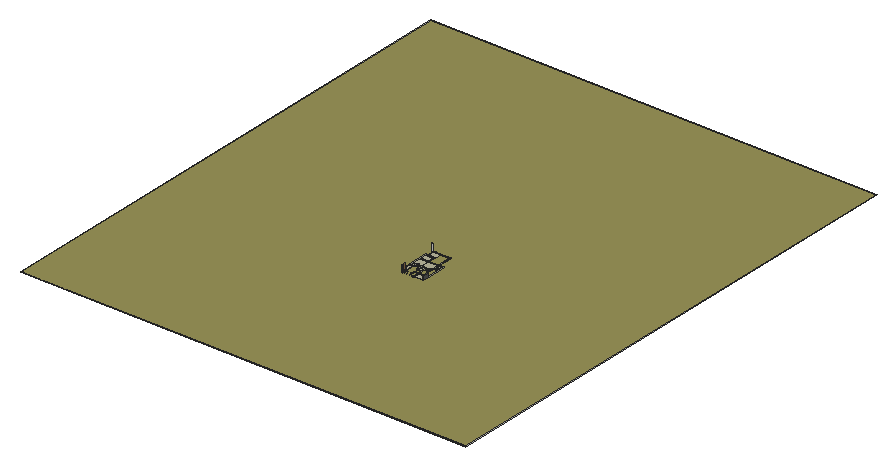
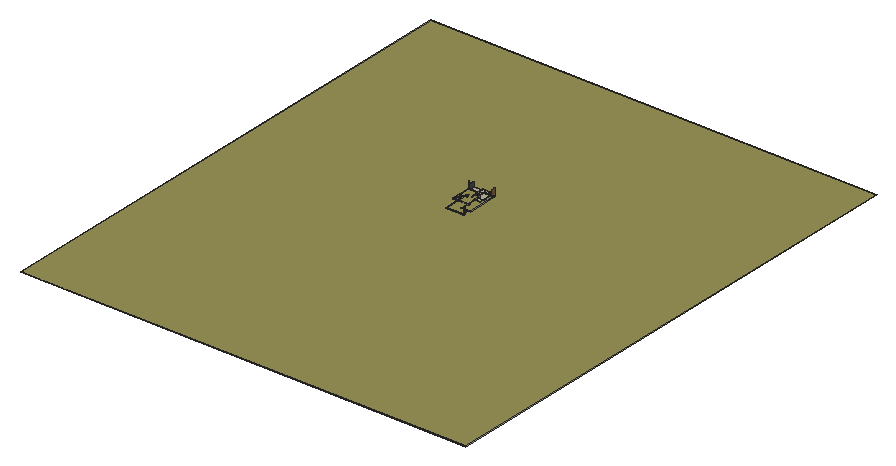
# SketchUp Ruby script. Lengths in inches.
U = 1.inch
M = Sketchup.active_model
def pt(a) = Geom::Point3d.new(a.map { |v| v * U })
def face(e, loops, mat)
  f = e.add_face(loops[0].map { |a| pt(a) })
  loops[1..].each { |l| e.add_face(l.map { |a| pt(a) }).erase! }
  f.material = f.back_material = mat if mat
  f
end
# faces: each face lists its corners as indices into pts; further lists are holes
def faces(e, pts, list, mat = nil) = list.each { |f| face(e, (f[0].is_a?(Array) ? f : [f]).map { |l| l.map { |i| pts[i] } }, mat) }
# xy, xz, yz: faces in a plane at the given z, y or x. An outline is a flat list of corners, or four numbers for a rectangle; further outlines are holes
def ring(l) = l.size == 4 ? [[l[0], l[1]], [l[2], l[1]], [l[2], l[3]], [l[0], l[3]]] : l.each_slice(2).to_a
def flat(e, list, mat, &to3) = list.each { |f| face(e, (f[0].is_a?(Array) ? f : [f]).map { |l| ring(l).map { |u, v| to3.(u, v) } }, mat) }
def xy(e, z, list, mat = nil) = flat(e, list, mat) { |x, y| [x, y, z] }
def xz(e, y, list, mat = nil) = flat(e, list, mat) { |x, z| [x, y, z] }
def yz(e, x, list, mat = nil) = flat(e, list, mat) { |y, z| [x, y, z] }
def lines(e, pts, list) = list.each { |a, b| e.add_line(pt(pts[a]), pt(pts[b])) }
# prism: a flat outline (further loops are holes) pulled along v
def prism(e, loops, v, mat = nil)
  f = face(e, loops, mat); d = Geom::Vector3d.new(v.map { |x| x * U })
  f.pushpull(f.normal.samedirection?(d) ? d.length : -d.length)
end
def box(e, o, s, mat = nil) = prism(e, [[o, [o[0] + s[0], o[1], o[2]], [o[0] + s[0], o[1] + s[1], o[2]], [o[0], o[1] + s[1], o[2]]]], [0, 0, s[2]], mat)
def at(x, y, z, deg = 0) = Geom::Transformation.translation(pt([x, y, z])) * Geom::Transformation.rotation(ORIGIN, Z_AXIS, deg.degrees)
def axes(o, x, y, z) = Geom::Transformation.new([*x, 0, *y, 0, *z, 0, *pt(o).to_a, 1])
def part(name) = M.definitions.add(name)
# library, detail: a bought-in or finely detailed component or shape, given as its bounding box
def library(name, o, s) = part(name).tap { |d| box(d.entities, o, s) }
def detail(e, o, s) = box(e.add_group.entities, o, s)
def put(e, d, t, mat = nil) = e.add_instance(d, t).tap { |i| i.material = mat if mat }
def group(e, t, mat = nil) = e.add_group.tap { |g| g.transformation = t; g.material = mat if mat }.entities
root = M.entities
M.materials.add("Concrete_04_1K").color = [184, 181, 156]
M.materials.add("M06_Steel_Smoke").color = [86, 86, 86]
M.materials.add("Plywood_01_1K").color = [125, 96, 64]
M.materials.add("Soil_04_1K").color = [152, 146, 88]
M.materials.add("Wood_Floor_01_1K").color = [146, 111, 76]
xy(root,9,[[4480,3552.7,4489,3625.01],[4489,3552.7,4621.87,3625.01],[4621.87,3552.7,4625.87,3625.01],[4625.87,3552.7,4682.8125,3635.25],[4682.8125,3552.7,4700.3125,3635.25],
  [4462.07,3564.51,4462.07,3609.04,4472.4375,3609.04,4472.4375,3625.01,4480,3625.01,4480,3564.51],[4700.3125,3566.51,4861.07,3666.98],[4861.07,3566.51,4874.8125,3666.98],[4430.07,3609.04,4472.4375,3609.04,4472.4375,3639.11,4480,3639.11,4480,3645.11,4429.38,3645.11,4429.38,3639.11,4430.07,3639.11],[4472.4375,3625.01,4480,3639.11],
  [4480,3625.01,4489,3805.79],[4489,3625.01,4489,3805.79,4591.8125,3805.79,4591.8125,3746.01,4621.87,3746.01,4621.87,3625.01],[4621.87,3625.01,4625.87,3631.25],[4621.87,3631.25,4625.87,3635.25],[4621.87,3635.25,4625.87,3666.98],
  [4625.87,3635.25,4682.8125,3666.98],[4682.8125,3635.25,4700.3125,3666.98],[4420.38,3639.11,4429.38,3645.11],[4420.38,3645.11,4429.38,3800.79],[4429.38,3645.11,4480,3800.79],
  [4621.87,3666.98,4625.87,3670.98],[4625.87,3666.98,4686.8125,3670.98],[4686.8125,3666.98,4690.8125,3670.98],[4690.8125,3666.98,4870.8125,3670.98],[4870.8125,3666.98,4874.8125,3670.98],
  [4621.87,3670.98,4625.87,3750.01],[4625.87,3670.98,4686.8125,3750.01],[4686.8125,3670.98,4690.8125,3833.04],[4870.8125,3670.98,4874.8125,3833.04],[4591.8125,3746.01,4595.8125,3750.01],
  [4595.8125,3746.01,4621.87,3750.01],[4591.8125,3750.01,4595.8125,3766.09],[4595.8125,3750.01,4686.8125,3833.04],[4591.8125,3766.09,4595.8125,3833.04],[4420.38,3800.79,4429.38,3809.79],
  [4429.38,3800.79,4480,3809.79],[4480,3805.79,4489,3809.79],[4489,3805.79,4591.8125,3809.79],[4420.38,3809.79,4489,3869.04],[4489,3809.79,4591.8125,3869.04],
  [4591.8125,3833.04,4595.8125,3869.04],[4595.8125,3833.04,4778.8125,3869.04],[4778.8125,3833.04,4784.8125,3923.04],[4865.8125,3833.04,4874.8125,3923.04],[4420.38,3869.04,4489,3878.04],
  [4489,3869.04,4591.8125,3878.04],[4723.125,3869.04,4729.125,3878.04],[4729.125,3869.04,4778.8125,3878.04],[4420.38,3878.04,4586.8125,4049.04],[4586.8125,3878.04,4595.8125,4049.04],
  [4595.8125,3878.04,4595.8125,4049.04,4769.8125,4049.04,4769.8125,4040.04,4778.8125,4040.04,4778.8125,3878.04],[4778.8125,3923.04,4784.8125,3929.04],[4784.8125,3923.04,4865.8125,3929.04],[4865.8125,3923.04,4874.8125,3929.04],[4778.8125,3929.04,4784.8125,3977.04],
  [4784.8125,3929.04,4865.8125,3977.04],[4865.8125,3929.04,4874.8125,3977.04],[4778.8125,3977.04,4784.8125,3983.04],[4784.8125,3977.04,4865.8125,3983.04],[4865.8125,3977.04,4874.8125,3983.04],
  [4778.8125,3983.04,4784.8125,4040.04],[4784.8125,3983.04,4865.8125,4040.04],[4865.8125,3983.04,4874.8125,4040.04],[4769.8125,4040.04,4778.8125,4049.04],[4778.8125,4040.04,4865.8125,4049.04],
  [4865.8125,4040.04,4874.8125,4049.04],[4420.38,4049.04,4586.8125,4058.04],[4586.8125,4049.04,4595.8125,4058.04],[4769.8125,4049.04,4778.8125,4058.04],[4420.38,4058.04,4586.8125,4176.04],
  [4769.8125,4058.04,4778.8125,4328.04],[4420.38,4176.04,4586.8125,4193.04],[4454.8125,4193.04,4463.8125,4202.04],[4463.8125,4193.04,4586.8125,4202.04],[4454.8125,4202.04,4463.8125,4328.04],
  [4463.8125,4202.04,4591.8125,4328.04],[4454.8125,4328.04,4463.8125,4337.04],[4463.8125,4328.04,4591.8125,4337.04],[4591.8125,4328.04,4769.8125,4337.04],[4769.8125,4328.04,4778.8125,4337.04]],"Concrete_04_1K")
xz(root,3552.7,[[4480,9,4700.3125,15]],"Plywood_01_1K")
xz(root,3564.51,[[4462.07,9,4480,124.125]],"Wood_Floor_01_1K")
xz(root,3566.51,[[4861.07,9,4874.8125,81.29]],"M06_Steel_Smoke")
xz(root,3609.04,[[4462.07,9,4472.4375,15]],"Concrete_04_1K")
xz(root,3609.04,[[4430.07,9,4462.07,15]],"Plywood_01_1K")
xz(root,3639.11,[[4472.4375,9,4480,15]],"Concrete_04_1K")
xz(root,3639.11,[[4420.38,9,4430.07,15]],"Plywood_01_1K")
xz(root,3645.11,[[4429.38,9,4480,15]],"Concrete_04_1K")
xz(root,3666.98,[[4625.87,9,4682.8125,9,4695.7,15,4625.87,15],[4682.8125,9,4700.3125,9,4700.3125,15,4695.7,15],[4700.3125,9,4861.07,15],[4861.07,9,4874.8125,15]],"Concrete_04_1K")
xz(root,3670.98,[[4625.87,9,4686.8125,15],[4690.8125,9,4870.8125,15]],"Concrete_04_1K")
xz(root,3746.01,[[4591.8125,9,4595.8125,15],[4595.8125,9,4621.87,15]],"Concrete_04_1K")
xz(root,3750.01,[[4595.8125,9,4621.87,15],[4621.87,9,4625.87,15],[4625.87,9,4686.8125,15]],"Concrete_04_1K")
xz(root,3800.79,[[4429.38,9,4480,15]],"Concrete_04_1K")
xz(root,3805.79,[[4489,9,4591.8125,15]],"Concrete_04_1K")
xz(root,3833.04,[[4686.8125,9,4690.8125,15],[4690.8125,9,4778.8125,15],[4778.8125,9,4784.8125,15],[4865.8125,9,4870.8125,15]],"Concrete_04_1K")
xz(root,3869.04,[[4489,9,4591.8125,15],[4723.125,9,4729.125,15],[4729.125,9,4778.8125,15]],"Concrete_04_1K")
xz(root,3878.04,[[4489,9,4586.8125,15],[4586.8125,9,4591.8125,15],[4591.8125,9,4595.8125,15],[4723.125,9,4729.125,15],[4729.125,9,4778.8125,15]],"Concrete_04_1K")
xz(root,3977.04,[[4784.8125,9,4865.8125,15]],"Concrete_04_1K")
xz(root,4040.04,[[4769.8125,9,4778.8125,15],[4778.8125,9,4784.8125,15],[4784.8125,9,4865.8125,15]],"Concrete_04_1K")
xz(root,4049.04,[[4595.8125,9,4769.8125,15],[4778.8125,9,4874.8125,15]],"Concrete_04_1K")
xz(root,4193.04,[[4420.38,9,4454.8125,15],[4454.8125,9,4586.8125,15]],"Concrete_04_1K")
xz(root,4202.04,[[4463.8125,9,4586.8125,15],[4586.8125,9,4591.8125,15]],"Concrete_04_1K")
xz(root,4328.04,[[4463.8125,9,4591.8125,15],[4591.8125,9,4769.8125,15]],"Concrete_04_1K")
xz(root,4337.04,[[4454.8125,9,4778.8125,15]],"Concrete_04_1K")
yz(root,4420.38,[[3639.11,9,3809.79,15],[3809.79,9,4193.04,15]],"Concrete_04_1K")
yz(root,4429.38,[[3645.11,9,3800.79,15]],"Concrete_04_1K")
yz(root,4430.07,[[3609.04,9,3639.11,15]],"Plywood_01_1K")
yz(root,4454.8125,[[4193.04,9,4337.04,15]],"Concrete_04_1K")
yz(root,4462.07,[[3564.51,9,3564.51,124.125,3639.11,124.125,3639.11,15,3611.04,15,3611.04,41.8125,3609.04,41.8125,3609.04,40,3609.73,40,3609.73,16,3609.04,16,3609.04,9]],"Wood_Floor_01_1K")
yz(root,4463.8125,[[4202.04,9,4328.04,15]],"Concrete_04_1K")
yz(root,4472.4375,[[3609.04,9,3639.11,15]],"Concrete_04_1K")
yz(root,4480,[[3564.51,9,3639.11,15],[3645.11,9,3800.79,15]],"Concrete_04_1K")
yz(root,4480,[[3552.7,9,3564.51,15]],"Wood_Floor_01_1K")
yz(root,4489,[[3625.01,9,3805.79,9,3805.79,15,3608.64,15],[3809.79,9,3869.04,15]],"Concrete_04_1K")
yz(root,4586.8125,[[3878.04,9,4049.04,15],[4058.04,9,4193.04,15]],"Concrete_04_1K")
yz(root,4591.8125,[[3750.54,9,3805.79,15],[3809.79,9,3833.04,15]],"Concrete_04_1K")
yz(root,4595.8125,[[3750.01,9,3833.04,15],[3833.04,9,3869.04,15],[3878.04,9,4049.04,15]],"Concrete_04_1K")
yz(root,4621.87,[[3625.01,9,3608.64,15,3631.25,15,3631.25,9],[3631.25,9,3635.25,15],[3635.25,9,3666.98,15],[3666.98,9,3670.98,15],[3670.98,9,3746.01,15]],"Concrete_04_1K")
yz(root,4625.87,[[3635.25,9,3666.98,15],[3670.98,9,3750.01,15]],"Concrete_04_1K")
yz(root,4686.8125,[[3670.98,9,3750.01,15],[3750.01,9,3833.04,15]],"Concrete_04_1K")
yz(root,4690.8125,[[3670.98,9,3833.04,15]],"Concrete_04_1K")
yz(root,4700.3125,[[3566.51,9,3666.98,9,3666.98,15]],"Concrete_04_1K")
yz(root,4700.3125,[[3552.7,9,3566.51,9,3666.98,15,3552.7,15]],"Plywood_01_1K")
yz(root,4769.8125,[[4049.04,9,4058.04,15],[4058.04,9,4328.04,15]],"Concrete_04_1K")
yz(root,4778.8125,[[3833.04,9,3869.04,15],[3869.04,9,3878.04,15],[3878.04,9,3923.04,15],[3923.04,9,3929.04,15],[3929.04,9,3977.04,15],
  [3977.04,9,3983.04,15],[3983.04,9,4040.04,15],[4049.04,9,4337.04,15]],"Concrete_04_1K")
yz(root,4784.8125,[[3833.04,9,3923.04,15],[3923.04,9,3929.04,15],[3929.04,9,3977.04,15],[3983.04,9,4040.04,15]],"Concrete_04_1K")
yz(root,4861.07,[[3566.51,9,3566.51,81.29,3660.98,81.29,3660.98,111,3666.98,111,3666.98,15],[3566.51,9,3666.98,15,3666.98,9]],"M06_Steel_Smoke")
yz(root,4865.8125,[[3833.04,9,3923.04,15],[3929.04,9,3977.04,15],[3983.04,9,4040.04,15]],"Concrete_04_1K")
yz(root,4870.8125,[[3670.98,9,3833.04,15]],"Concrete_04_1K")
yz(root,4874.8125,[[3666.98,9,4049.04,15]],"Concrete_04_1K")
yz(root,4874.8125,[[3566.51,9,3666.98,9,3666.98,141,3660.98,141,3660.98,81.29,3566.51,81.29]],"M06_Steel_Smoke")
p = [[4621.87,3625.01,9],[4489,3625.01,9],[4489,3608.64,15],[4498.625,3608.64,15],[4546.625,3608.64,15],[4553.37,3608.64,15],
  [4601.37,3608.64,15],[4621.87,3608.64,15],[4682.8125,3666.98,9],[4682.8125,3635.25,9],[4695.7,3635.25,15],[4695.7,3666.98,15],
  [4591.8125,3750.01,9],[4591.8125,3750.01,15],[4595.8125,4058.04,9],[4595.8125,4058.04,15]]
faces(root,p,[[0,1,2,3,4,5,6,7],[8,9,10,11]],"Concrete_04_1K")
lines(root,p,[[12,13],[14,15]])
g1 = group(root,at(4291.75,3492.5625,0))
xy(g1,0,[[-4291.75,-3492.5625,4244.8125,6338.625]])
xy(g1,9,[[-4291.75,-3492.5625,4244.8125,6338.625]],"Soil_04_1K")
xz(g1,-3492.5625,[[-4291.75,0,4244.8125,9]])
xz(g1,6338.625,[[-4291.75,0,4244.8125,9]])
yz(g1,-4291.75,[[-3492.5625,0,6338.625,9]])
yz(g1,4244.8125,[[-3492.5625,0,6338.625,9]])
g2 = group(root,at(4420.38,4328.04,141))
box(g2,[0,0,-132],[9,9,132])
g3 = group(root,at(4700.3125,3566.51,9),"Concrete_04_1K")
p = [[160.76,0,0],[160.76,100.47,6],[0,100.47,6],[0,0,0]]
faces(g3,p,[[0,1,2,3]])
